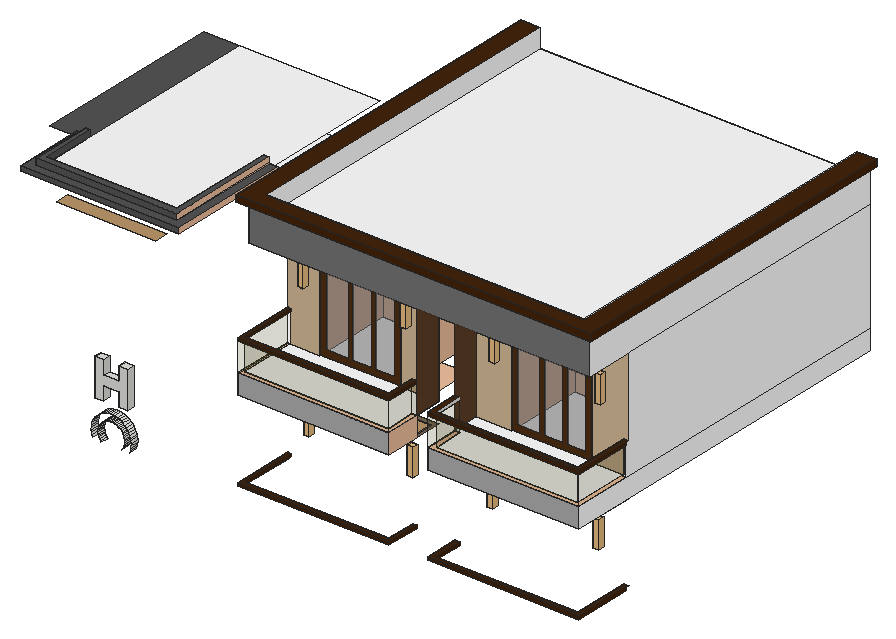
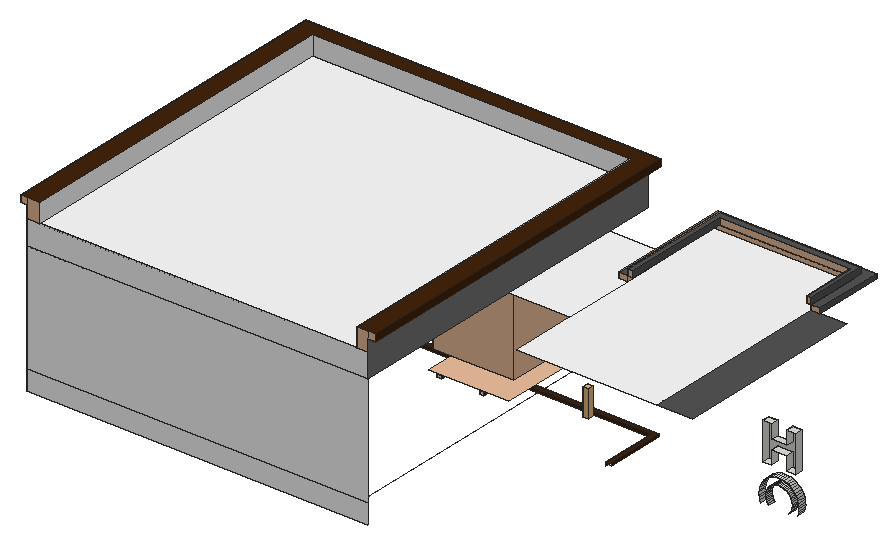
# SketchUp Ruby script. Lengths in inches.
U = 1.inch
M = Sketchup.active_model
def pt(a) = Geom::Point3d.new(a.map { |v| v * U })
def face(e, loops, mat)
  f = e.add_face(loops[0].map { |a| pt(a) })
  loops[1..].each { |l| e.add_face(l.map { |a| pt(a) }).erase! }
  f.material = f.back_material = mat if mat
  f
end
# faces: each face lists its corners as indices into pts; further lists are holes
def faces(e, pts, list, mat = nil) = list.each { |f| face(e, (f[0].is_a?(Array) ? f : [f]).map { |l| l.map { |i| pts[i] } }, mat) }
# xy, xz, yz: faces in a plane at the given z, y or x. An outline is a flat list of corners, or four numbers for a rectangle; further outlines are holes
def ring(l) = l.size == 4 ? [[l[0], l[1]], [l[2], l[1]], [l[2], l[3]], [l[0], l[3]]] : l.each_slice(2).to_a
def flat(e, list, mat, &to3) = list.each { |f| face(e, (f[0].is_a?(Array) ? f : [f]).map { |l| ring(l).map { |u, v| to3.(u, v) } }, mat) }
def xy(e, z, list, mat = nil) = flat(e, list, mat) { |x, y| [x, y, z] }
def xz(e, y, list, mat = nil) = flat(e, list, mat) { |x, z| [x, y, z] }
def yz(e, x, list, mat = nil) = flat(e, list, mat) { |y, z| [x, y, z] }
def lines(e, pts, list) = list.each { |a, b| e.add_line(pt(pts[a]), pt(pts[b])) }
# prism: a flat outline (further loops are holes) pulled along v
def prism(e, loops, v, mat = nil)
  f = face(e, loops, mat); d = Geom::Vector3d.new(v.map { |x| x * U })
  f.pushpull(f.normal.samedirection?(d) ? d.length : -d.length)
end
def box(e, o, s, mat = nil) = prism(e, [[o, [o[0] + s[0], o[1], o[2]], [o[0] + s[0], o[1] + s[1], o[2]], [o[0], o[1] + s[1], o[2]]]], [0, 0, s[2]], mat)
def at(x, y, z, deg = 0) = Geom::Transformation.translation(pt([x, y, z])) * Geom::Transformation.rotation(ORIGIN, Z_AXIS, deg.degrees)
def axes(o, x, y, z) = Geom::Transformation.new([*x, 0, *y, 0, *z, 0, *pt(o).to_a, 1])
def part(name) = M.definitions.add(name)
# library, detail: a bought-in or finely detailed component or shape, given as its bounding box
def library(name, o, s) = part(name).tap { |d| box(d.entities, o, s) }
def detail(e, o, s) = box(e.add_group.entities, o, s)
def put(e, d, t, mat = nil) = e.add_instance(d, t).tap { |i| i.material = mat if mat }
def group(e, t, mat = nil) = e.add_group.tap { |g| g.transformation = t; g.material = mat if mat }.entities
root = M.entities
M.materials.add("Generic").color = [68, 36, 11]
M.materials.add("Generic\#1").color = [84, 84, 84]
M.materials.add("Generic\#10").color = [214, 187, 153]
M.materials.add("Generic\#13").color = [239, 192, 158]
M.materials.add("Generic\#3").color = [117, 117, 117]
M.materials.add("Generic\#4").color = [186, 149, 106]
M.materials.add("Generic\#5").color = [175, 175, 175]
M.materials.add("Generic\#6").color = [117, 101, 81]
M.materials.add("[Color M00]").color = [255, 255, 255]
M.materials.add("[Translucent Glass Dark Green]").color = [86, 83, 28]
M.materials["[Translucent Glass Dark Green]"].alpha = 0.11
M.materials.add("[Translucent Glass Gray]1").color = [127, 127, 127]
M.materials["[Translucent Glass Gray]1"].alpha = 0.3
M.materials.add("[Wood Bamboo]").color = [81, 48, 19]
M.materials.add("[Wood Floor]").color = [91, 62, 36]
M.materials["[Wood Floor]"].alpha = 0.99
c1 = library("Wall Lamp 298 005",[-4.37,-9,-20.45],[8.74,9.125,40.9])
c2 = library("Tlon Light 450 Ceiling 152 006",[-8.86,-8.86,-3.78],[17.72,17.72,3.56])
c3 = part("Group\#13")
xy(c3.entities,0,[[0,0,104.75,3]])
xy(c3.entities,142.8125,[[0,0,104.75,3]])
xz(c3.entities,0,[[8.08,8.08,37.11,134.73],[42.61,8.08,67.14,134.73],[72.39,8.08,96.67,134.73]],"[Translucent Glass Gray]1")
xz(c3.entities,0,[[[0,0,104.75,142.8125],[8.08,8.08,37.11,134.73],[42.61,8.08,67.14,134.73],[72.39,8.08,96.67,134.73]]],"[Wood Bamboo]")
xz(c3.entities,3,[[0,0,104.75,142.8125]],"[Translucent Glass Gray]1")
yz(c3.entities,0,[[0,0,3,142.8125]])
yz(c3.entities,104.75,[[0,0,3,142.8125]])
xy(root,704.1875,[[404,60.0625,404,136.9375,408.8125,136.9375,408.8125,66.0625,596,66.0625,596,104.5,601.0625,104.5,601.0625,60.0625],[650.9375,60.0625,650.9375,104.5,657.6875,104.5,657.6875,66.0625,842,66.0625,842,136.9375,848,136.9375,848,60.0625]])
xy(root,708.0625,[[404,60.0625,601.0625,60.0625,601.0625,104.5,596,104.5,596,66.0625,408.8125,66.0625,408.8125,140.75,404,140.75],[650.9375,60.0625,848,60.0625,848,140.75,842,140.75,842,66.0625,657.6875,66.0625,657.6875,104.5,650.9375,104.5]],"Generic")
xy(root,735.92,[[210.88,68.3125,222.88,78.3125],[242.57,68.3125,254.57,78.3125]])
xy(root,753.92,[[222.88,68.3125,242.57,78.3125]])
xy(root,765.92,[[222.88,68.3125,242.57,78.3125]])
xy(root,783.92,[[210.88,68.3125,222.88,78.3125],[242.57,68.3125,254.57,78.3125]])
xy(root,808.9375,[[452.52,140.75,557.27,243.1875],[696.14,140.75,800.89,243.1875]],"Generic\#13")
xy(root,809.875,[[[404,60.0625,601.0625,140.75],[408.26,64.32,596.81,132.68]],[[650.9375,60.0625,848,140.75],[655.77,64.89,843.17,132.11]]],"Generic\#6")
xy(root,811.1875,[[408.26,64.32,596.81,132.68],[655.77,64.89,843.17,132.11]],"Generic\#4")
xy(root,835.625,[[404,60.0625,404,140.75,408.0625,140.75,408.0625,66.0625,595.3125,66.0625,595.3125,104.5,601.0625,104.5,601.0625,60.0625],[650.9375,60.0625,650.9375,104.5,657.95,104.5,657.95,66.0625,842,66.0625,842,136.9375,848,136.9375,848,60.0625]],"Generic\#13")
xy(root,835.625,[[408.0625,66.0625,595.3125,66.0625,595.3125,104.5,601.0625,104.5,601.0625,140.75,551.52,140.75,551.52,243.1875,446.77,243.1875,446.77,140.75,408.0625,140.75],[657.95,66.0625,842,66.0625,842,140.75,800.89,140.75,800.89,243.1875,696.14,243.1875,696.14,140.75,650.9375,140.75,650.9375,104.5,657.95,104.5]],"[Color M00]")
xy(root,873.0625,[[404,60.0625,404,140.75,408.0625,140.75,408.0625,66.0625,595.3125,66.0625,595.3125,104.5,601.0625,104.5,601.0625,60.0625],[650.9375,60.0625,650.9375,104.5,657.95,104.5,657.95,66.0625,842,66.0625,842,136.9375,848,136.9375,848,60.0625]])
xy(root,877.1875,[[404,60.0625,601.0625,60.0625,601.0625,104.5,595.3125,104.5,595.3125,66.0625,408.0625,66.0625,408.0625,140.75,404,140.75],[650.9375,60.0625,848,60.0625,848,140.75,842,140.75,842,66.0625,657.95,66.0625,657.95,104.5,650.9375,104.5]],"Generic")
xy(root,952.73,[[168.02,60.4375,297.35,78.3125]],"Generic\#4")
xy(root,979.625,[[94.0625,140.75,141.125,391.6875]],"Generic\#1")
xy(root,979.625,[[129.6875,49,129.6875,60.4375,133.5625,60.4375,133.5625,70.1875,141.125,70.1875,141.125,60.4375,335.6875,60.4375,335.6875,49],[129.6875,60.4375,133.5625,70.1875],[141.125,60.4375,324.25,69.5],[324.25,60.4375,335.6875,140.75],[129.6875,70.1875,141.125,79.9375],
  [601.0625,78.3125,650.9375,104.5],[129.6875,79.9375,141.125,140.75],[601.0625,104.5,601.0625,140.75,551.52,140.75,551.52,243.1875,446.77,243.1875,446.77,140.75,404,140.75,404,534.3125,848,534.3125,848,140.75,800.89,140.75,800.89,243.1875,696.14,243.1875,696.14,140.75,650.9375,140.75,650.9375,104.5],[324.25,140.75,335.6875,210.875]],"Generic\#13")
xy(root,979.625,[[[404,78.3125,404,140.75,446.77,140.75,446.77,243.1875,551.52,243.1875,551.52,140.75,601.0625,140.75,601.0625,78.3125],[414.42,88.74,590.64,130.33]],[650.9375,78.3125,650.9375,140.75,661.15,140.75,661.15,88.53,837.78,88.53,837.78,140.75,848,140.75,848,78.3125],[661.15,126.72,661.15,140.75,696.14,140.75,696.14,243.1875,800.89,243.1875,800.89,140.75,837.78,140.75,837.78,126.72]],"Generic\#6")
xy(root,979.625,[[141.125,69.5,324.25,391.6875],[335.6875,140.75,404,140.75,404,304.75,324.25,304.75,324.25,210.875,335.6875,210.875]],"[Color M00]")
xy(root,986.25,[[129.6875,49,335.6875,49,335.6875,210.875,324.25,210.875,324.25,59.97,141.125,59.97,141.125,140.75,129.6875,140.75]],"Generic\#1")
xy(root,986.25,[[141.125,59.97,324.25,69.5],[141.125,69.5,147.375,140.75],[316.75,69.5,324.25,210.875]],"Generic\#13")
xy(root,988.3125,[[661.15,88.53,837.78,126.72],[414.42,88.74,590.64,130.33]],"Generic\#4")
xy(root,994.0625,[[141.125,59.97,324.25,59.97,324.25,210.875,316.75,210.875,316.75,69.5,147.375,69.5,147.375,140.75,141.125,140.75]],"Generic\#1")
xy(root,1011.3125,[[418.25,89.375,831,534.3125]],"[Color M00]")
xy(root,1027.125,[[393.6875,69.6875,393.6875,534.3125,404,534.3125,404,78.3125,848,78.3125,848,534.3125,856,534.3125,856,69.6875]],"Generic")
xy(root,1035.6875,[[393.6875,69.6875,856,69.6875,856,534.3125,831,534.3125,831,89.375,418.25,89.375,418.25,534.3125,393.6875,534.3125]],"Generic")
xz(root,49,[[129.6875,979.625,335.6875,986.25]],"Generic\#1")
xz(root,59.97,[[141.125,986.25,324.25,994.0625]],"Generic\#1")
xz(root,60.0625,[[404,704.1875,601.0625,708.0625],[650.9375,704.1875,848,708.0625],[404,873.0625,601.0625,877.1875],[650.9375,873.0625,848,877.1875]],"Generic")
xz(root,60.0625,[[404,809.875,601.0625,835.625],[650.9375,809.875,848,835.625]],"Generic\#5")
xz(root,60.0625,[[404,835.625,601.0625,873.0625],[650.9375,835.625,848,873.0625]],"[Translucent Glass Dark Green]")
xz(root,64.32,[[408.26,809.875,596.81,811.1875]])
xz(root,64.89,[[655.77,809.875,843.17,811.1875]])
xz(root,66.0625,[[408.0625,873.0625,595.3125,877.1875],[657.95,873.0625,842,877.1875]])
xz(root,66.0625,[[408.8125,704.1875,596,708.0625],[657.6875,704.1875,842,708.0625]],"Generic")
xz(root,66.0625,[[408.0625,835.625,595.3125,873.0625],[657.95,835.625,842,873.0625]],"[Translucent Glass Dark Green]")
xz(root,68.3125,[[210.88,735.92,222.88,735.92,222.88,753.92,242.57,753.92,242.57,735.92,254.57,735.92,254.57,783.92,242.57,783.92,242.57,765.92,222.88,765.92,222.88,783.92,210.88,783.92]])
xz(root,69.5,[[141.125,979.625,324.25,986.25],[147.375,986.25,316.75,994.0625]],"Generic\#13")
xz(root,69.6875,[[393.6875,1027.125,856,1035.6875]],"Generic")
xz(root,78.3125,[[404,979.625,848,1027.125]],"Generic\#3")
xz(root,88.53,[[661.15,979.625,837.78,988.3125]])
xz(root,88.74,[[414.42,979.625,590.64,988.3125]])
xz(root,89.375,[[418.25,1011.3125,831,1035.6875]],"[Color M00]")
xz(root,104.5,[[596,704.1875,601.0625,708.0625],[650.9375,704.1875,657.6875,708.0625],[595.3125,873.0625,601.0625,877.1875],[650.9375,873.0625,657.95,877.1875]])
xz(root,104.5,[[595.3125,835.625,601.0625,873.0625],[650.9375,835.625,657.95,873.0625]],"[Translucent Glass Dark Green]")
xz(root,126.72,[[661.15,979.625,837.78,988.3125]],"Generic\#6")
xz(root,130.33,[[414.42,979.625,590.64,988.3125]],"Generic\#6")
xz(root,132.11,[[655.77,809.875,843.17,811.1875]],"Generic\#6")
xz(root,132.68,[[408.26,809.875,440,811.1875],[440,809.875,596.81,811.1875]],"Generic\#6")
xz(root,140.75,[[408.0625,835.625,446.77,835.625,446.77,979.625,404,979.625,404,877.1875,408.0625,877.1875],[551.52,835.625,601.0625,979.625],[650.9375,835.625,696.14,979.625],[800.89,835.625,842,835.625,842,877.1875,848,877.1875,848,979.625,800.89,979.625]],"Generic\#10")
xz(root,140.75,[[129.6875,979.625,141.125,986.25],[141.125,986.25,147.375,994.0625]],"Generic\#13")
xz(root,210.875,[[324.25,979.625,335.6875,986.25],[316.75,986.25,324.25,994.0625]],"Generic\#13")
xz(root,243.1875,[[446.77,835.625,551.52,979.625],[696.14,835.625,800.89,979.625]],"Generic\#13")
xz(root,534.3125,[[404,1011.3125,418.25,1035.6875],[831,1011.3125,848,1035.6875],[393.6875,1027.125,404,1035.6875],[848,1027.125,856,1035.6875]],"Generic\#13")
xz(root,534.3125,[[404,809.875,848,835.625],[404,835.625,848,979.625],[404,979.625,848,1011.3125]],"[Color M00]")
yz(root,129.6875,[[49,979.625,140.75,986.25]],"Generic\#1")
yz(root,141.125,[[59.97,986.25,140.75,994.0625]],"Generic\#1")
yz(root,141.125,[[69.5,979.625,140.75,986.25]],"Generic\#13")
yz(root,147.375,[[69.5,986.25,140.75,994.0625]],"Generic\#1")
yz(root,210.88,[[68.3125,735.92,78.3125,783.92]])
yz(root,222.88,[[68.3125,735.92,78.3125,753.92],[68.3125,765.92,78.3125,783.92]])
yz(root,242.57,[[68.3125,735.92,78.3125,753.92],[68.3125,765.92,78.3125,783.92]])
yz(root,254.57,[[68.3125,735.92,78.3125,783.92]])
yz(root,316.75,[[69.5,986.25,210.875,994.0625]],"Generic\#1")
yz(root,324.25,[[69.5,979.625,210.875,986.25],[59.97,986.25,210.875,994.0625]],"Generic\#13")
yz(root,335.6875,[[49,979.625,210.875,986.25]],"Generic\#13")
yz(root,393.6875,[[69.6875,1027.125,534.3125,1035.6875]],"Generic")
yz(root,404,[[60.0625,704.1875,136.9375,708.0625],[60.0625,873.0625,140.75,877.1875]],"Generic")
yz(root,404,[[60.0625,809.875,140.75,835.625]],"Generic\#13")
yz(root,404,[[78.3125,979.625,534.3125,1027.125]],"Generic\#3")
yz(root,404,[[60.0625,835.625,140.75,873.0625]],"[Translucent Glass Dark Green]")
yz(root,408.0625,[[66.0625,873.0625,140.75,877.1875]],"Generic")
yz(root,408.0625,[[66.0625,835.625,140.75,873.0625]],"[Translucent Glass Dark Green]")
yz(root,408.26,[[64.32,809.875,132.68,811.1875]],"Generic\#6")
yz(root,408.8125,[[66.0625,704.1875,140.75,708.0625]],"Generic")
yz(root,414.42,[[88.74,979.625,130.33,988.3125]],"Generic\#6")
yz(root,418.25,[[89.375,1011.3125,534.3125,1035.6875]],"[Color M00]")
yz(root,446.77,[[140.75,835.625,243.1875,979.625]],"Generic\#13")
yz(root,551.52,[[140.75,835.625,243.1875,979.625]],"Generic\#13")
yz(root,590.64,[[88.74,979.625,104.5,988.3125],[104.5,979.625,130.33,988.3125]],"Generic\#6")
yz(root,595.3125,[[66.0625,873.0625,104.5,877.1875]],"Generic")
yz(root,595.3125,[[66.0625,835.625,104.5,873.0625]],"[Translucent Glass Dark Green]")
yz(root,596,[[66.0625,704.1875,104.5,708.0625]],"Generic")
yz(root,596.81,[[64.32,809.875,104.5,811.1875],[104.5,809.875,132.68,811.1875]],"Generic\#6")
yz(root,601.0625,[[60.0625,704.1875,104.5,708.0625],[60.0625,873.0625,104.5,877.1875]],"Generic")
yz(root,601.0625,[[60.0625,809.875,104.5,835.625]],"Generic\#13")
yz(root,601.0625,[[60.0625,835.625,104.5,873.0625]],"[Translucent Glass Dark Green]")
yz(root,601.0625,[[104.5,835.625,140.75,979.625]],"[Wood Floor]")
yz(root,650.9375,[[60.0625,704.1875,104.5,708.0625],[60.0625,873.0625,104.5,877.1875]],"Generic")
yz(root,650.9375,[[60.0625,809.875,104.5,835.625]],"Generic\#13")
yz(root,650.9375,[[60.0625,835.625,104.5,873.0625]],"[Translucent Glass Dark Green]")
yz(root,650.9375,[[104.5,835.625,140.75,979.625]],"[Wood Floor]")
yz(root,655.77,[[64.89,809.875,132.11,811.1875]],"Generic\#6")
yz(root,657.6875,[[66.0625,704.1875,104.5,708.0625]],"Generic")
yz(root,657.95,[[66.0625,873.0625,104.5,877.1875]])
yz(root,657.95,[[66.0625,835.625,104.5,873.0625]],"[Translucent Glass Dark Green]")
yz(root,661.15,[[88.53,979.625,126.72,988.3125]],"Generic\#6")
yz(root,696.14,[[140.75,835.625,243.1875,979.625]],"Generic\#13")
yz(root,800.89,[[140.75,835.625,243.1875,979.625]],"Generic\#13")
yz(root,831,[[89.375,1011.3125,534.3125,1035.6875]],"[Color M00]")
yz(root,837.78,[[88.53,979.625,126.72,988.3125]],"Generic\#6")
yz(root,842,[[66.0625,704.1875,140.75,708.0625],[66.0625,873.0625,140.75,877.1875]],"Generic")
yz(root,842,[[66.0625,835.625,140.75,873.0625]],"[Translucent Glass Dark Green]")
yz(root,843.17,[[64.89,809.875,132.11,811.1875]],"Generic\#6")
yz(root,848,[[60.0625,704.1875,136.9375,708.0625],[60.0625,873.0625,136.9375,877.1875]],"Generic")
yz(root,848,[[60.0625,809.875,534.3125,835.625],[136.9375,835.625,534.3125,835.625,534.3125,979.625,140.75,979.625,140.75,877.1875,136.9375,877.1875],[78.3125,979.625,534.3125,1027.125]],"[Color M00]")
yz(root,848,[[60.0625,835.625,136.9375,873.0625]],"[Translucent Glass Dark Green]")
yz(root,856,[[69.6875,1027.125,534.3125,1035.6875]],"Generic")
p = [[219.58,78.3125,686.84],[218.41,78.3125,688.39],[218.41,68.3125,688.39],[219.58,68.3125,686.84],[256.55,78.3125,687.44],[257.58,78.3125,690.17],
  [257.58,68.3125,690.17],[256.55,68.3125,687.44],[247.61,78.3125,689.29],[246.54,78.3125,687.68],[246.54,68.3125,687.68],[247.61,68.3125,689.29],
  [217.42,78.3125,690.05],[217.42,68.3125,690.05],[207.51,78.3125,691.43],[208.4,78.3125,688.65],[208.4,68.3125,688.65],[207.51,68.3125,691.43],
  [248.5,78.3125,691.01],[248.5,68.3125,691.01],[216.625,78.3125,691.8125],[216.625,68.3125,691.8125],[258.3,78.3125,693],[258.3,68.3125,693],
  [249.18,78.3125,692.82],[249.18,68.3125,692.82],[206.93,78.3125,694.3],[206.93,68.3125,694.3],[216.03,78.3125,693.66],[216.03,68.3125,693.66],
  [249.66,78.3125,694.69],[249.66,68.3125,694.69],[258.7,78.3125,695.9],[258.7,68.3125,695.9],[215.65,78.3125,695.55],[215.65,68.3125,695.55],
  [206.68,78.3125,697.21],[206.68,68.3125,697.21],[249.92,78.3125,696.61],[249.92,68.3125,696.61],[215.48,78.3125,697.48],[215.48,68.3125,697.48],
  [258.78,78.3125,698.82],[258.78,68.3125,698.82],[249.97,78.3125,698.55],[249.97,68.3125,698.55],[206.75,78.3125,700.13],[206.75,68.3125,700.13],
  [215.53,78.3125,699.41],[215.53,68.3125,699.41],[249.8,78.3125,700.47],[249.8,68.3125,700.47],[258.52,78.3125,701.73],[258.52,68.3125,701.73],
  [215.8,78.3125,701.33],[215.8,68.3125,701.33],[207.15,78.3125,703.02],[207.15,68.3125,703.02],[249.42,78.3125,702.37],[249.42,68.3125,702.37],
  [216.27,78.3125,703.21],[216.27,68.3125,703.21],[257.95,78.3125,704.59],[257.95,68.3125,704.59],[248.83,78.3125,704.21],[248.83,68.3125,704.21],
  [207.875,78.3125,705.86],[207.875,68.3125,705.86],[216.96,78.3125,705.01],[216.96,68.3125,705.01],[248.03,78.3125,705.98],[248.03,68.3125,705.98],
  [257.05,78.3125,707.375],[257.05,68.3125,707.375],[217.84,78.3125,706.74],[217.84,68.3125,706.74],[208.91,78.3125,708.59],[208.91,68.3125,708.59],
  [247.05,78.3125,707.64],[247.05,68.3125,707.64],[218.91,78.3125,708.35],[218.91,68.3125,708.35],[255.85,78.3125,710.04],[255.85,68.3125,710.04],
  [245.88,78.3125,709.18],[245.88,68.3125,709.18],[220.16,78.3125,709.83],[220.16,68.3125,709.83],[210.24,78.3125,711.19],[210.24,68.3125,711.19],
  [244.54,78.3125,710.58],[244.54,68.3125,710.58],[221.56,78.3125,711.16],[221.56,68.3125,711.16],[254.36,78.3125,712.55],[254.36,68.3125,712.55],
  [243.0625,78.3125,711.83],[243.0625,68.3125,711.83],[211.86,78.3125,713.625],[211.86,68.3125,713.625],[223.1,78.3125,712.33],[223.1,68.3125,712.33],
  [241.45,78.3125,712.9],[241.45,68.3125,712.9],[224.76,78.3125,713.32],[224.76,68.3125,713.32],[252.59,78.3125,714.88],[252.59,68.3125,714.88],
  [239.73,78.3125,713.78],[239.73,68.3125,713.78],[226.53,78.3125,714.11],[226.53,68.3125,714.11],[213.74,78.3125,715.86],[213.74,68.3125,715.86],
  [237.92,78.3125,714.47],[237.92,68.3125,714.47],[228.37,78.3125,714.71],[228.37,68.3125,714.71],[236.05,78.3125,714.94],[236.05,68.3125,714.94],
  [230.27,78.3125,715.09],[230.27,68.3125,715.09],[234.13,78.3125,715.21],[234.13,68.3125,715.21],[250.58,78.3125,717],[250.58,68.3125,717],
  [232.19,78.3125,715.26],[232.19,68.3125,715.26],[215.86,78.3125,717.88],[215.86,68.3125,717.88],[248.34,78.3125,718.88],[248.34,68.3125,718.88],
  [218.1875,78.3125,719.64],[218.1875,68.3125,719.64],[245.91,78.3125,720.5],[245.91,68.3125,720.5],[220.7,78.3125,721.13],[220.7,68.3125,721.13],
  [243.3,78.3125,721.83],[243.3,68.3125,721.83],[223.36,78.3125,722.33],[223.36,68.3125,722.33],[240.57,78.3125,722.87],[240.57,68.3125,722.87],
  [226.15,78.3125,723.23],[226.15,68.3125,723.23],[237.74,78.3125,723.59],[237.74,68.3125,723.59],[229.01,78.3125,723.81],[229.01,68.3125,723.81],
  [234.84,78.3125,723.99],[234.84,68.3125,723.99],[231.92,78.3125,724.0625],[231.92,68.3125,724.0625],[440,136.9375,809.875],[440,140.75,809.875],
  [812,136.9375,809.875],[812,140.75,809.875],[404,78.3125,1027.125],[404,78.3125,1033.125],[812,515.9375,809.875],[440,515.9375,809.875]]
faces(root,p,[[0,1,2,3],[4,5,6,7],[8,9,10,11],[1,12,13,2],[14,15,16,17],[18,8,11,19],[12,20,21,13],[5,22,23,6],
  [24,18,19,25],[26,14,17,27],[20,28,29,21],[30,24,25,31],[22,32,33,23],[28,34,35,29],[36,26,27,37],[38,30,31,39],
  [34,40,41,35],[32,42,43,33],[44,38,39,45],[46,36,37,47],[40,48,49,41],[50,44,45,51],[42,52,53,43],[48,54,55,49],
  [56,46,47,57],[58,50,51,59],[54,60,61,55],[52,62,63,53],[64,58,59,65],[66,56,57,67],[60,68,69,61],[70,64,65,71],
  [62,72,73,63],[68,74,75,69],[76,66,67,77],[78,70,71,79],[74,80,81,75],[72,82,83,73],[84,78,79,85],[80,86,87,81],
  [88,76,77,89],[90,84,85,91],[86,92,93,87],[82,94,95,83],[96,90,91,97],[98,88,89,99],[92,100,101,93],[102,96,97,103],
  [100,104,105,101],[94,106,107,95],[108,102,103,109],[104,110,111,105],[112,98,99,113],[114,108,109,115],[110,116,117,111],[118,114,115,119],
  [116,120,121,117],[122,118,119,123],[106,124,125,107],[120,126,127,121],[126,122,123,127],[128,112,113,129],[124,130,131,125],[132,128,129,133],
  [130,134,135,131],[136,132,133,137],[134,138,139,135],[140,136,137,141],[138,142,143,139],[144,140,141,145],[142,146,147,143],[148,144,145,149],
  [146,150,151,147],[152,148,149,153],[150,152,153,151]])
lines(root,p,[[154,155],[156,157],[158,159],[157,160],[155,161]])
put(root,c1,axes([574.69,134.14,763.81],[0.8568,0,0],[0,0.8568,0],[0,0,0.8568]))
put(root,c1,axes([440.07,134.14,763.81],[0.8568,0,0],[0,0.8568,0],[0,0,0.8568]))
put(root,c1,axes([679.44,134.14,763.81],[0.8568,0,0],[0,0.8568,0],[0,0,0.8568]))
put(root,c1,axes([816.88,134.14,763.81],[0.8568,0,0],[0,0.8568,0],[0,0,0.8568]))
put(root,c2,at(820.2,94.66,812.35))
put(root,c2,at(676.08,94.66,812.35))
put(root,c2,at(569.64,94.66,812.35))
put(root,c2,at(438.51,94.66,812.35))
put(root,c3,at(696.14,140.75,836.8125))
put(root,c3,at(446.77,140.75,836.8125))
put(root,c1,axes([432.32,134.14,934.18],[0.8568,0,0],[0,0.8568,0],[0,0,0.8568]))
put(root,c1,axes([565.76,134.14,934.18],[0.8568,0,0],[0,0.8568,0],[0,0,0.8568]))
put(root,c1,axes([681.32,134.14,934.18],[0.8568,0,0],[0,0.8568,0],[0,0,0.8568]))
put(root,c1,axes([819.32,134.14,934.18],[0.8568,0,0],[0,0.8568,0],[0,0,0.8568]))
put(root,c2,at(432.9,115.39,990.66))
put(root,c2,at(570.09,115.39,990.66))
put(root,c2,at(687.64,110.33,990.66))
put(root,c2,at(813.26,110.33,990.66))
put(root,c2,at(432.9,115.39,992.1))
